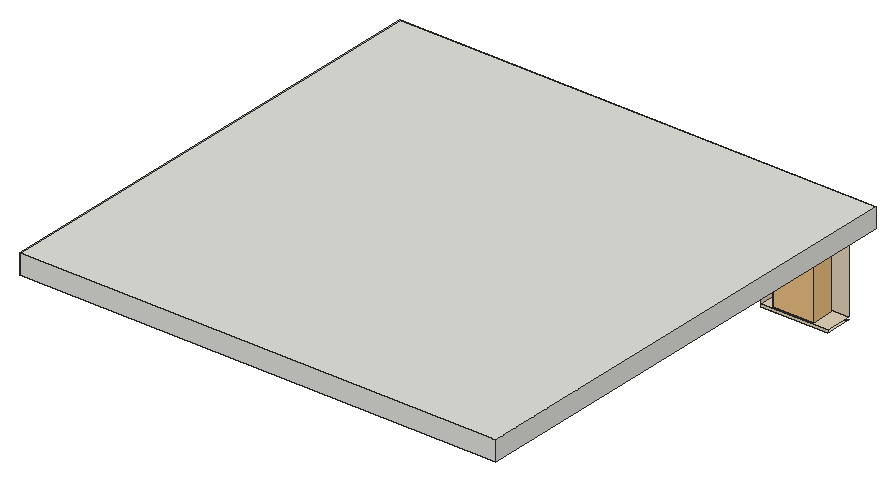
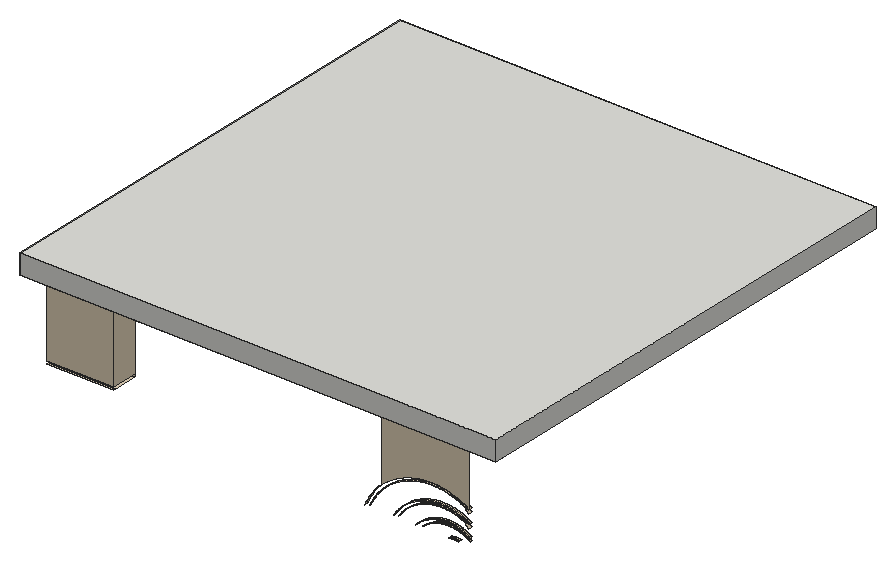
# SketchUp Ruby script. Lengths in inches.
U = 1.inch
M = Sketchup.active_model
def pt(a) = Geom::Point3d.new(a.map { |v| v * U })
def face(e, loops, mat)
  f = e.add_face(loops[0].map { |a| pt(a) })
  loops[1..].each { |l| e.add_face(l.map { |a| pt(a) }).erase! }
  f.material = f.back_material = mat if mat
  f
end
# faces: each face lists its corners as indices into pts; further lists are holes
def faces(e, pts, list, mat = nil) = list.each { |f| face(e, (f[0].is_a?(Array) ? f : [f]).map { |l| l.map { |i| pts[i] } }, mat) }
# xy, xz, yz: faces in a plane at the given z, y or x. An outline is a flat list of corners, or four numbers for a rectangle; further outlines are holes
def ring(l) = l.size == 4 ? [[l[0], l[1]], [l[2], l[1]], [l[2], l[3]], [l[0], l[3]]] : l.each_slice(2).to_a
def flat(e, list, mat, &to3) = list.each { |f| face(e, (f[0].is_a?(Array) ? f : [f]).map { |l| ring(l).map { |u, v| to3.(u, v) } }, mat) }
def xy(e, z, list, mat = nil) = flat(e, list, mat) { |x, y| [x, y, z] }
def xz(e, y, list, mat = nil) = flat(e, list, mat) { |x, z| [x, y, z] }
def yz(e, x, list, mat = nil) = flat(e, list, mat) { |y, z| [x, y, z] }
def lines(e, pts, list) = list.each { |a, b| e.add_line(pt(pts[a]), pt(pts[b])) }
# prism: a flat outline (further loops are holes) pulled along v
def prism(e, loops, v, mat = nil)
  f = face(e, loops, mat); d = Geom::Vector3d.new(v.map { |x| x * U })
  f.pushpull(f.normal.samedirection?(d) ? d.length : -d.length)
end
def box(e, o, s, mat = nil) = prism(e, [[o, [o[0] + s[0], o[1], o[2]], [o[0] + s[0], o[1] + s[1], o[2]], [o[0], o[1] + s[1], o[2]]]], [0, 0, s[2]], mat)
def at(x, y, z, deg = 0) = Geom::Transformation.translation(pt([x, y, z])) * Geom::Transformation.rotation(ORIGIN, Z_AXIS, deg.degrees)
def axes(o, x, y, z) = Geom::Transformation.new([*x, 0, *y, 0, *z, 0, *pt(o).to_a, 1])
def part(name) = M.definitions.add(name)
# library, detail: a bought-in or finely detailed component or shape, given as its bounding box
def library(name, o, s) = part(name).tap { |d| box(d.entities, o, s) }
def detail(e, o, s) = box(e.add_group.entities, o, s)
def put(e, d, t, mat = nil) = e.add_instance(d, t).tap { |i| i.material = mat if mat }
def group(e, t, mat = nil) = e.add_group.tap { |g| g.transformation = t; g.material = mat if mat }.entities
root = M.entities
M.materials.add("Teddy_Brim").color = [225, 210, 185]
M.materials.add("[Color M00]1").color = [255, 255, 255]
c1 = library("Telephone 194 013",[-6.23,-3.22,0.01],[12.47,6.44,15])
c2 = part("Group\#159")
detail(c2.entities,[2.83,2.83,12.39],[3.25,3.25,0.24])
g1 = group(c2.entities,at(3.45,3.45,12.51))
xy(g1,0,[[1,0,0.74,0.03,0.5,0.13,0.29,0.29,0.13,0.5,0.03,0.74,0,1,0.03,1.25,0.13,1.49,0.29,1.7,0.5,1.86,0.74,1.96,1,1.99,1.25,1.96,1.49,1.86,1.7,1.7,1.86,1.49,1.96,1.25,1.99,1,1.96,0.74,1.86,0.5,1.7,0.29,1.49,0.13,1.25,0.03]],"[Color M00]1")
xy(root,89.28,[[15.7,138.5,15.89,139.5],[16.26,138.5,16.44,139.5]],"Teddy_Brim")
xy(root,92.11,[[18.02,138.5,18.28,139]],"Teddy_Brim")
xy(root,93.19,[[18.1,138.5,18.37,139.5],[18.37,138.5,18.64,139.5]],"Teddy_Brim")
xy(root,93.61,[[119.125,131.5,139.5,138.79]],"Teddy_Brim")
xy(root,94.39,[[119.125,131.5,139.5,139.5]],"Teddy_Brim")
xy(root,96.38,[[19.92,138.5,20.25,139]],"Teddy_Brim")
xy(root,97.38,[[19.91,138.5,20.26,139.5]],"Teddy_Brim")
xy(root,101.36,[[22.9375,138.5,23.38,139]],"Teddy_Brim")
xy(root,102.36,[[22.93,138.5,23.39,139.5]],"Teddy_Brim")
xy(root,118,[[115.125,131.5,119.125,131.5,119.125,139.5,139.5,139.5,139.5,144,4.5,144,4.5,139.5,8.5,139.5,8.5,137.5,11.5,137.5,11.5,139.5,115.125,139.5]],"Teddy_Brim")
xz(root,131.5,[[119.125,93.61,139.5,94.39]],"Teddy_Brim")
xz(root,139.5,[[119.125,94.39,139.5,118],[37.98,96.48,37.98,118,11.5,118,11.5,99,12.3,99.48,12.7,99.71,13.52,100.13,13.94,100.33,14.37,100.52,14.79,100.71,15.22,100.88,16.1,101.2,16.98,101.48,17.43,101.6,17.875,101.72,18.33,101.83,18.78,101.92,19.24,102.01,19.69,102.09,20.15,102.16,20.61,102.22,21.08,102.26,21.54,102.3,22,102.33,22.46,102.35,22.93,102.36,23.39,102.36,23.86,102.35,24.32,102.33,24.78,102.3,25.25,102.25,25.71,102.2,26.17,102.14,26.625,102.07,27.08,101.99,27.54,101.9,28.44,101.7,28.89,101.58,29.34,101.45,29.78,101.3125,30.22,101.16,30.66,101.01,31.52,100.67,31.95,100.48,32.37,100.29,32.79,100.09,33.2,99.88,33.61,99.66,34.01,99.43,34.41,99.19,34.72,99,34.81,98.95,35.19,98.69,35.58,98.43,35.96,98.16,36.33,97.88,36.69,97.6,37.05,97.3,37.4,97,37.75,96.69]],"Teddy_Brim")
yz(root,119.125,[[131.5,94.39,139.5,118]],"Teddy_Brim")
p = [[14.78,139.5,89.19],[14.6,139.5,89.16],[14.6,138.5,89.16],[14.78,138.5,89.19],[14.97,139.5,89.22],[14.97,138.5,89.22],
  [15.15,139.5,89.24],[15.15,138.5,89.24],[15.33,139.5,89.26],[15.33,138.5,89.26],[17,139.5,89.24],[16.8125,139.5,89.26],
  [16.8125,138.5,89.26],[17,138.5,89.24],[17.18,139.5,89.22],[17.18,138.5,89.22],[17.36,139.5,89.19],[17.36,138.5,89.19],
  [17.55,139.5,89.16],[17.55,138.5,89.16],[25.625,138.5,89.4],[25.625,139,89.4],[25.82,139,89.24],[25.82,138.5,89.24],
  [41.81,138.5,89.6],[41.81,139,89.6],[42,139,89.2],[42,138.5,89.2],[43.1,139.5,89.19],[42.91,139.5,89.62],
  [42.91,138.5,89.62],[43.1,138.5,89.19],[15.52,139.5,89.27],[15.52,138.5,89.27],[15.7,139.5,89.28],[15.7,138.5,89.28],
  [16.07,139.5,89.29],[15.89,139.5,89.28],[15.89,138.5,89.28],[16.07,138.5,89.29],[16.26,139.5,89.28],[16.26,138.5,89.28],
  [16.63,139.5,89.27],[16.44,139.5,89.28],[16.44,138.5,89.28],[16.63,138.5,89.27],[27.56,139.5,89.26],[27.37,139.5,89.45],
  [27.37,138.5,89.45],[27.56,138.5,89.26],[25.42,138.5,89.57],[25.42,139,89.57],[33.01,138.5,89.67],[33.01,139,89.67],
  [33.19,139,89.4],[33.19,138.5,89.4],[34.41,139.5,89.36],[34.22,139.5,89.66],[34.22,138.5,89.66],[34.41,138.5,89.36],
  [27.18,139.5,89.64],[27.18,138.5,89.64],[25.22,138.5,89.72],[25.22,139,89.72],[26.99,139.5,89.83],[26.99,138.5,89.83],
  [41.61,138.5,90],[41.61,139,90],[42.71,139.5,90.04],[42.71,138.5,90.04],[25.01,138.5,89.88],[25.01,139,89.88],
  [32.8125,138.5,89.94],[32.8125,139,89.94],[34.02,139.5,89.95],[34.02,138.5,89.95],[26.79,139.5,90.02],[26.79,138.5,90.02],
  [24.8,138.5,90.03],[24.8,139,90.03],[32.61,138.5,90.21],[32.61,139,90.21],[24.59,138.5,90.17],[24.59,139,90.17],
  [26.58,139.5,90.19],[26.58,138.5,90.19],[33.82,139.5,90.24],[33.82,138.5,90.24],[41.41,138.5,90.39],[41.41,139,90.39],
  [42.51,139.5,90.45],[42.51,138.5,90.45],[11.5,138.9,90.05],[11.5,139,90.05],[11.7,139,90.1875],[11.7,138.5,90.1875],
  [11.5,138.5,90.05],[11.92,139,90.33],[11.92,138.5,90.33],[24.375,138.5,90.31],[24.375,139,90.31],[26.375,139.5,90.37],
  [26.375,138.5,90.37],[32.41,138.5,90.47],[32.41,139,90.47],[33.62,139.5,90.53],[33.62,138.5,90.53],[12.14,139,90.46],
  [12.14,138.5,90.46],[24.15,138.5,90.45],[24.15,139,90.45],[23.93,138.5,90.57],[23.93,139,90.57],[26.17,139.5,90.54],
  [26.17,138.5,90.54],[41.2,138.5,90.78],[41.2,139,90.78],[12.36,139,90.59],[12.36,138.5,90.59],[25.95,139.5,90.71],
  [25.95,138.5,90.71],[32.2,138.5,90.73],[32.2,139,90.73],[33.41,139.5,90.81],[33.41,138.5,90.81],[42.29,139.5,90.86],
  [42.29,138.5,90.86],[12.58,139,90.71],[12.58,138.5,90.71],[23.71,138.5,90.7],[23.71,139,90.7],[12.8125,139,90.83],
  [12.8125,138.5,90.83],[23.48,138.5,90.82],[23.48,139,90.82],[25.73,139.5,90.87],[25.73,138.5,90.87],[31.98,138.5,90.98],
  [31.98,139,90.98],[13.04,139,90.95],[13.04,138.5,90.95],[23.25,138.5,90.93],[23.25,139,90.93],[33.1875,139.5,91.09],
  [33.1875,138.5,91.09],[40.98,138.5,91.16],[40.98,139,91.16],[13.28,139,91.06],[13.28,138.5,91.06],[23.02,138.5,91.04],
  [23.02,139,91.04],[25.51,139.5,91.02],[25.51,138.5,91.02],[42.07,139.5,91.27],[42.07,138.5,91.27],[11.72,139.5,91.15],
  [11.5,139.5,91],[11.5,138.9,91],[11.5,138.5,91],[11.72,138.5,91.15],[22.78,138.5,91.15],[22.78,139,91.15],
  [25.29,139.5,91.17],[25.29,138.5,91.17],[31.76,138.5,91.23],[31.76,139,91.23],[13.51,139,91.16],[13.51,138.5,91.16],
  [22.54,138.5,91.25],[22.54,139,91.25],[32.96,139.5,91.37],[32.96,138.5,91.37],[11.95,139.5,91.3],[11.95,138.5,91.3],
  [13.75,139,91.26],[13.75,138.5,91.26],[22.3,138.5,91.34],[22.3,139,91.34],[25.06,139.5,91.32],[25.06,138.5,91.32],
  [31.53,138.5,91.47],[31.53,139,91.47],[40.75,138.5,91.54],[40.75,139,91.54],[12.18,139.5,91.44],[12.18,138.5,91.44],
  [13.99,139,91.35],[13.99,138.5,91.35],[22.0625,138.5,91.43],[22.0625,139,91.43],[24.83,139.5,91.46],[24.83,138.5,91.46],
  [41.84,139.5,91.67],[41.84,138.5,91.67],[12.42,139.5,91.58],[12.42,138.5,91.58],[14.23,139,91.44],[14.23,138.5,91.44],
  [14.47,139,91.52],[14.47,138.5,91.52],[21.82,138.5,91.52],[21.82,139,91.52],[32.74,139.5,91.64],[32.74,138.5,91.64],
  [14.72,139,91.6],[14.72,138.5,91.6],[21.57,138.5,91.59],[21.57,139,91.59],[24.59,139.5,91.6],[24.59,138.5,91.6],
  [31.3,138.5,91.71],[31.3,139,91.71],[40.51,138.5,91.92],[40.51,139,91.92],[12.65,139.5,91.71],[12.65,138.5,91.71],
  [14.97,139,91.67],[14.97,138.5,91.67],[21.33,138.5,91.67],[21.33,139,91.67],[24.36,139.5,91.73],[24.36,138.5,91.73],
  [32.5,139.5,91.9],[32.5,138.5,91.9],[12.89,139.5,91.83],[12.89,138.5,91.83],[15.22,139,91.74],[15.22,138.5,91.74],
  [15.47,139,91.8],[15.47,138.5,91.8],[20.83,138.5,91.8],[20.83,139,91.8],[21.08,139,91.73],[21.08,138.5,91.73],
  [24.12,139.5,91.85],[24.12,138.5,91.85],[31.07,138.5,91.94],[31.07,139,91.94],[41.6,139.5,92.07],[41.6,138.5,92.07],
  [13.14,139.5,91.96],[13.14,138.5,91.96],[15.72,139,91.86],[15.72,138.5,91.86],[20.58,138.5,91.85],[20.58,139,91.85],
  [15.97,139,91.91],[15.97,138.5,91.91],[16.22,139,91.95],[16.22,138.5,91.95],[19.81,138.5,91.99],[19.81,139,91.99],
  [20.07,139,91.95],[20.07,138.5,91.95],[20.32,139,91.9],[20.32,138.5,91.9],[23.87,139.5,91.97],[23.87,138.5,91.97],
  [30.82,138.5,92.17],[30.82,139,92.17],[32.26,139.5,92.16],[32.26,138.5,92.16],[40.26,138.5,92.29],[40.26,139,92.29],
  [13.38,139.5,92.07],[13.38,138.5,92.07],[16.48,139,91.99],[16.48,138.5,91.99],[16.73,139,92.03],[16.73,138.5,92.03],
  [16.99,139,92.05],[16.99,138.5,92.05],[19.3,138.5,92.05],[19.3,139,92.05],[19.56,139,92.02],[19.56,138.5,92.02],
  [23.63,139.5,92.09],[23.63,138.5,92.09],[13.63,139.5,92.18],[13.63,138.5,92.18],[17.25,139,92.08],[17.25,138.5,92.08],
  [17.5,139,92.09],[17.5,138.5,92.09],[17.76,139,92.1],[17.76,138.5,92.1],[18.02,139,92.11],[18.02,138.5,92.11],
  [18.28,138.5,92.11],[18.28,139,92.11],[18.53,139,92.1],[18.53,138.5,92.1],[18.79,139,92.09],[18.79,138.5,92.09],
  [19.05,139,92.07],[19.05,138.5,92.07],[23.38,139.5,92.2],[23.38,138.5,92.2],[41.35,139.5,92.46],[41.35,138.5,92.46],
  [13.88,139.5,92.29],[13.88,138.5,92.29],[23.13,139.5,92.3],[23.13,138.5,92.3],[30.58,138.5,92.4],[30.58,139,92.4],
  [32.01,139.5,92.41],[32.01,138.5,92.41],[14.13,139.5,92.38],[14.13,138.5,92.38],[22.875,139.5,92.4],[22.875,138.5,92.4],
  [40.01,138.5,92.65],[40.01,139,92.65],[14.38,139.5,92.48],[14.38,138.5,92.48],[22.62,139.5,92.49],[22.62,138.5,92.49],
  [30.33,138.5,92.61],[30.33,139,92.61],[31.76,139.5,92.66],[31.76,138.5,92.66],[14.64,139.5,92.57],[14.64,138.5,92.57],
  [22.37,139.5,92.58],[22.37,138.5,92.58],[41.09,139.5,92.85],[41.09,138.5,92.85],[14.9,139.5,92.65],[14.9,138.5,92.65],
  [15.16,139.5,92.73],[15.16,138.5,92.73],[22.11,139.5,92.66],[22.11,138.5,92.66],[30.07,138.5,92.83],[30.07,139,92.83],
  [39.75,138.5,93.01],[39.75,139,93.01],[15.42,139.5,92.8],[15.42,138.5,92.8],[21.85,139.5,92.74],[21.59,139.5,92.81],
  [21.59,138.5,92.81],[21.85,138.5,92.74],[31.51,139.5,92.91],[31.51,138.5,92.91],[15.68,139.5,92.86],[15.68,138.5,92.86],
  [21.32,139.5,92.87],[21.32,138.5,92.87],[29.8125,138.5,93.04],[29.8125,139,93.04],[40.82,139.5,93.23],[40.82,138.5,93.23],
  [15.95,139.5,92.92],[15.95,138.5,92.92],[16.21,139.5,92.97],[16.21,138.5,92.97],[21.06,139.5,92.93],[20.79,139.5,92.98],
  [20.79,138.5,92.98],[21.06,138.5,92.93],[31.24,139.5,93.14],[31.24,138.5,93.14],[16.48,139.5,93.02],[16.48,138.5,93.02],
  [16.75,139.5,93.06],[16.75,138.5,93.06],[20.53,139.5,93.03],[20.26,139.5,93.07],[20.26,138.5,93.07],[20.53,138.5,93.03],
  [29.55,138.5,93.24],[29.55,139,93.24],[39.48,138.5,93.36],[39.48,139,93.36],[17.02,139.5,93.1],[17.02,138.5,93.1],
  [17.29,139.5,93.13],[17.29,138.5,93.13],[17.56,139.5,93.15],[17.56,138.5,93.15],[19.72,139.5,93.13],[19.45,139.5,93.16],
  [19.45,138.5,93.16],[19.72,138.5,93.13],[19.99,139.5,93.11],[19.99,138.5,93.11],[30.98,139.5,93.375],[30.98,138.5,93.375],
  [17.83,139.5,93.17],[17.83,138.5,93.17],[18.1,139.5,93.19],[18.1,138.5,93.19],[18.91,139.5,93.1875],[18.64,139.5,93.19],
  [18.64,138.5,93.19],[18.91,138.5,93.1875],[19.18,139.5,93.18],[19.18,138.5,93.18],[29.28,138.5,93.43],[29.28,139,93.43],
  [40.55,139.5,93.6],[40.55,138.5,93.6],[29.01,138.5,93.625],[29.01,139,93.625],[30.71,139.5,93.6],[30.71,138.5,93.6],
  [39.21,138.5,93.7],[39.21,139,93.7],[28.73,138.5,93.81],[28.73,139,93.81],[30.43,139.5,93.82],[30.43,138.5,93.82],
  [40.27,139.5,93.97],[40.27,138.5,93.97],[38.92,138.5,94.05],[38.92,139,94.05],[28.45,138.5,93.99],[28.45,139,93.99],
  [30.15,139.5,94.04],[30.15,138.5,94.04],[11.5,139.5,93.86],[12.5,139.5,94.42],[12.5,139,94.42],[12.5,138.5,94.42],
  [11.5,138.5,93.86],[11.5,138.9,93.86],[28.17,138.5,94.16],[28.17,139,94.16],[29.86,139.5,94.25],[29.86,138.5,94.25],
  [38.63,138.5,94.38],[38.63,139,94.38],[39.98,139.5,94.34],[39.98,138.5,94.34],[27.88,138.5,94.33],[27.88,139,94.33],
  [29.57,139.5,94.45],[29.57,138.5,94.45],[27.59,138.5,94.49],[27.59,139,94.49],[39.68,139.5,94.69],[39.68,138.5,94.69],
  [12.59,139,94.47],[12.59,138.5,94.47],[38.34,138.5,94.71],[38.34,139,94.71],[12.89,139,94.63],[12.89,138.5,94.63],
  [27.29,138.5,94.65],[27.29,139,94.65],[29.28,139.5,94.65],[29.28,138.5,94.65],[13.18,139,94.78],[13.18,138.5,94.78],
  [27,138.5,94.79],[27,139,94.79],[28.98,139.5,94.84],[28.98,138.5,94.84],[38.03,138.5,95.03],[38.03,139,95.03],
  [39.38,139.5,95.04],[39.38,138.5,95.04],[13.48,139,94.92],[13.48,138.5,94.92],[26.7,138.5,94.9375],[26.7,139,94.9375],
  [28.68,139.5,95.02],[28.68,138.5,95.02],[13.79,139,95.06],[13.79,138.5,95.06],[26.39,138.5,95.07],[26.39,139,95.07],
  [11.81,139.5,95.18],[11.5,139.5,95],[11.5,138.9,95],[11.5,138.5,95],[11.81,138.5,95.18],[28.375,139.5,95.2],
  [28.375,138.5,95.2],[37.72,138.5,95.34],[37.72,139,95.34],[39.07,139.5,95.39],[39.07,138.5,95.39],[14.09,139,95.1875],
  [14.09,138.5,95.1875],[26.09,138.5,95.2],[26.09,139,95.2],[12.11,139.5,95.35],[12.11,138.5,95.35],[14.4,139,95.3125],
  [14.4,138.5,95.3125],[25.78,138.5,95.32],[25.78,139,95.32],[28.0625,139.5,95.37],[28.0625,138.5,95.37],[14.71,139,95.43],
  [14.71,138.5,95.43],[25.47,138.5,95.44],[25.47,139,95.44],[37.4,138.5,95.65],[37.4,139,95.65],[12.43,139.5,95.52],
  [12.43,138.5,95.52],[15.03,139,95.54],[15.03,138.5,95.54],[25.15,138.5,95.55],[25.15,139,95.55],[27.75,139.5,95.54],
  [27.75,138.5,95.54],[38.75,139.5,95.72],[38.75,138.5,95.72],[12.74,139.5,95.67],[12.74,138.5,95.67],[15.34,139,95.64],
  [15.34,138.5,95.64],[27.43,139.5,95.69],[27.43,138.5,95.69],[15.66,139,95.74],[15.66,138.5,95.74],[24.84,138.5,95.65],
  [24.84,139,95.65],[13.0625,139.5,95.83],[13.0625,138.5,95.83],[15.98,139,95.83],[15.98,138.5,95.83],[24.52,138.5,95.75],
  [24.52,139,95.75],[27.12,139.5,95.84],[27.12,138.5,95.84],[37.08,138.5,95.95],[37.08,139,95.95],[38.42,139.5,96.05],
  [38.42,138.5,96.05],[13.38,139.5,95.97],[13.38,138.5,95.97],[16.3,139,95.91],[16.3,138.5,95.91],[23.875,138.5,95.92],
  [23.875,139,95.92],[24.2,139,95.84],[24.2,138.5,95.84],[26.79,139.5,95.99],[26.79,138.5,95.99],[16.625,139,95.99],
  [16.625,138.5,95.99],[23.55,138.5,96],[23.55,139,96],[13.71,139.5,96.11],[13.71,138.5,96.11],[16.95,139,96.0625],
  [16.95,138.5,96.0625],[23.23,138.5,96.07],[23.23,139,96.07],[26.47,139.5,96.13],[26.47,138.5,96.13],[36.75,138.5,96.25],
  [36.75,139,96.25],[14.04,139.5,96.24],[14.04,138.5,96.24],[17.28,139,96.125],[17.28,138.5,96.125],[17.6,139,96.18],
  [17.6,138.5,96.18],[22.57,138.5,96.1875],[22.57,139,96.1875],[22.9,139,96.13],[22.9,138.5,96.13],[26.14,139.5,96.26],
  [26.14,138.5,96.26],[38.09,139.5,96.38],[38.09,138.5,96.38],[14.37,139.5,96.37],[14.37,138.5,96.37],[17.93,139,96.23],
  [17.93,138.5,96.23],[18.26,139,96.27],[18.26,138.5,96.27],[21.91,138.5,96.28],[21.91,139,96.28],[22.24,139,96.24],
  [22.24,138.5,96.24],[36.41,138.5,96.54],[36.41,139,96.54],[18.59,139,96.31],[18.59,138.5,96.31],[18.93,139,96.34],
  [18.93,138.5,96.34],[19.26,139,96.36],[19.26,138.5,96.36],[20.92,138.5,96.36],[20.92,139,96.36],[21.25,139,96.34],
  [21.25,138.5,96.34],[21.58,139,96.3125],[21.58,138.5,96.3125],[25.81,139.5,96.38],[25.81,138.5,96.38],[14.7,139.5,96.48],
  [14.7,138.5,96.48],[19.59,139,96.37],[19.59,138.5,96.37],[19.92,139,96.38],[19.92,138.5,96.38],[20.25,138.5,96.38],
  [20.25,139,96.38],[20.59,139,96.375],[20.59,138.5,96.375],[25.47,139.5,96.5],[25.47,138.5,96.5],[37.98,139.5,96.48],
  [37.75,139.5,96.69],[37.75,138.5,96.69],[15.04,139.5,96.6],[15.04,138.5,96.6],[25.14,139.5,96.61],[25.14,138.5,96.61],
  [36.07,138.5,96.82],[36.07,139,96.82],[15.38,139.5,96.7],[15.38,138.5,96.7],[24.8,139.5,96.71],[24.8,138.5,96.71],
  [15.72,139.5,96.8],[15.72,138.5,96.8],[24.46,139.5,96.81],[24.46,138.5,96.81],[37.4,139.5,97],[37.4,138.5,97],
  [16.06,139.5,96.88],[16.06,138.5,96.88],[24.11,139.5,96.89],[24.11,138.5,96.89],[35.72,138.5,97.09],[35.72,139,97.09],
  [16.4,139.5,96.97],[16.4,138.5,96.97],[23.77,139.5,96.98],[23.77,138.5,96.98],[16.75,139.5,97.04],[16.75,138.5,97.04],
  [17.1,139.5,97.11],[17.1,138.5,97.11],[23.42,139.5,97.05],[23.08,139.5,97.12],[23.08,138.5,97.12],[23.42,138.5,97.05],
  [37.05,139.5,97.3],[37.05,138.5,97.3],[17.45,139.5,97.17],[17.45,138.5,97.17],[22.73,139.5,97.17],[22.73,138.5,97.17],
  [35.36,138.5,97.35],[35.36,139,97.35],[17.8,139.5,97.22],[17.8,138.5,97.22],[18.15,139.5,97.27],[18.15,138.5,97.27],
  [22.38,139.5,97.23],[22.03,139.5,97.27],[22.03,138.5,97.27],[22.38,138.5,97.23],[18.5,139.5,97.3],[18.5,138.5,97.3],
  [18.85,139.5,97.33],[18.85,138.5,97.33],[19.2,139.5,97.36],[19.2,138.5,97.36],[21.32,139.5,97.34],[20.97,139.5,97.36],
  [20.97,138.5,97.36],[21.32,138.5,97.34],[21.68,139.5,97.31],[21.68,138.5,97.31],[36.69,139.5,97.6],[36.69,138.5,97.6],
  [19.56,139.5,97.37],[19.56,138.5,97.37],[19.91,139.5,97.38],[19.91,138.5,97.38],[20.62,139.5,97.375],[20.26,139.5,97.38],
  [20.26,138.5,97.38],[20.62,138.5,97.375],[35,138.5,97.61],[35,139,97.61],[34.64,138.5,97.86],[34.64,139,97.86],
  [36.33,139.5,97.88],[36.33,138.5,97.88],[11.5,139.5,97.85],[12.5,139.5,98.4375],[12.5,139,98.4375],[12.5,138.5,98.4375],
  [11.5,138.5,97.85],[11.5,138.9,97.85],[34.27,138.5,98.1],[34.27,139,98.1],[35.96,139.5,98.16],[35.96,138.5,98.16],
  [34.19,138.5,98.15],[34.19,139,98.15],[33.89,138.5,98.34],[33.89,139,98.34],[35.58,139.5,98.43],[35.58,138.5,98.43],
  [33.51,138.5,98.5625],[33.51,139,98.5625],[12.79,139,98.61],[12.79,138.5,98.61],[35.19,139.5,98.69],[35.19,138.5,98.69],
  [13.18,139,98.83],[13.18,138.5,98.83],[33.125,138.5,98.78],[33.125,139,98.78],[34.81,139.5,98.95],[34.81,138.5,98.95],
  [13.57,139,99.04],[13.57,138.5,99.04],[32.74,138.5,98.99],[32.74,139,98.99],[34.72,139.5,99],[34.72,138.5,99],
  [11.9,139.5,99.24],[11.5,139.5,99],[11.5,138.9,99],[11.5,138.5,99],[11.9,138.5,99.24],[13.97,139,99.23],
  [13.97,138.5,99.23],[32.34,138.5,99.19],[32.34,139,99.19],[34.41,139.5,99.19],[34.41,138.5,99.19],[12.3,139.5,99.48],
  [12.3,138.5,99.48],[14.36,139,99.43],[14.36,138.5,99.43],[31.94,138.5,99.39],[31.94,139,99.39],[34.01,139.5,99.43],
  [34.01,138.5,99.43],[14.77,139,99.61],[14.77,138.5,99.61],[31.54,138.5,99.57],[31.54,139,99.57],[33.61,139.5,99.66],
  [33.61,138.5,99.66],[12.7,139.5,99.71],[12.7,138.5,99.71],[15.18,139,99.78],[15.18,138.5,99.78],[31.13,138.5,99.75],
  [31.13,139,99.75],[13.11,139.5,99.92],[13.11,138.5,99.92],[30.72,138.5,99.91],[30.72,139,99.91],[33.2,139.5,99.88],
  [33.2,138.5,99.88],[15.59,139,99.95],[15.59,138.5,99.95],[13.52,139.5,100.13],[13.52,138.5,100.13],[16,139,100.1],
  [16,138.5,100.1],[30.3125,138.5,100.07],[30.3125,139,100.07],[32.79,139.5,100.09],[32.79,138.5,100.09],[13.94,139.5,100.33],
  [13.94,138.5,100.33],[16.42,139,100.25],[16.42,138.5,100.25],[29.89,138.5,100.22],[29.89,139,100.22],[32.37,139.5,100.29],
  [32.37,138.5,100.29],[16.84,139,100.39],[16.84,138.5,100.39],[29.47,138.5,100.36],[29.47,139,100.36],[14.37,139.5,100.52],
  [14.37,138.5,100.52],[31.95,139.5,100.48],[31.95,138.5,100.48],[17.26,139,100.52],[17.26,138.5,100.52],[29.05,138.5,100.49],
  [29.05,139,100.49],[14.79,139.5,100.71],[14.79,138.5,100.71],[17.6875,139,100.64],[17.6875,138.5,100.64],[28.625,138.5,100.61],
  [28.625,139,100.61],[31.52,139.5,100.67],[31.52,138.5,100.67],[18.12,139,100.75],[18.12,138.5,100.75],[28.2,138.5,100.73],
  [28.2,139,100.73],[15.22,139.5,100.88],[15.22,138.5,100.88],[18.55,139,100.85],[18.55,138.5,100.85],[27.77,138.5,100.83],
  [27.77,139,100.83],[31.09,139.5,100.84],[31.09,138.5,100.84],[27.33,138.5,100.93],[27.33,139,100.93],[30.66,139.5,101.01],
  [30.66,138.5,101.01],[15.66,139.5,101.04],[15.66,138.5,101.04],[18.98,139,100.94],[18.98,138.5,100.94],[19.42,139,101.03],
  [19.42,138.5,101.03],[26.9,138.5,101.01],[26.9,139,101.01],[16.1,139.5,101.2],[16.1,138.5,101.2],[19.85,139,101.1],
  [19.85,138.5,101.1],[26.46,138.5,101.09],[26.46,139,101.09],[30.22,139.5,101.16],[30.22,138.5,101.16],[20.29,139,101.17],
  [20.29,138.5,101.17],[26.03,138.5,101.15],[26.03,139,101.15],[16.54,139.5,101.34],[16.54,138.5,101.34],[20.73,139,101.22],
  [20.73,138.5,101.22],[21.17,139,101.27],[21.17,138.5,101.27],[25.15,138.5,101.26],[25.15,139,101.26],[25.59,139,101.21],
  [25.59,138.5,101.21],[29.78,139.5,101.3125],[29.78,138.5,101.3125],[16.98,139.5,101.48],[16.98,138.5,101.48],[21.61,139,101.31],
  [21.61,138.5,101.31],[22.05,139,101.33],[22.05,138.5,101.33],[22.49,139,101.35],[22.49,138.5,101.35],[23.38,138.5,101.36],
  [23.38,139,101.36],[23.82,139,101.35],[23.82,138.5,101.35],[24.26,139,101.33],[24.26,138.5,101.33],[24.71,139,101.3],
  [24.71,138.5,101.3],[29.34,139.5,101.45],[29.34,138.5,101.45],[22.9375,139,101.36],[22.9375,138.5,101.36],[28.89,139.5,101.58],
  [28.89,138.5,101.58],[17.43,139.5,101.6],[17.43,138.5,101.6],[17.875,139.5,101.72],[17.875,138.5,101.72],[28.44,139.5,101.7],
  [28.44,138.5,101.7],[18.33,139.5,101.83],[18.33,138.5,101.83],[27.99,139.5,101.8],[27.99,138.5,101.8],[18.78,139.5,101.92],
  [18.78,138.5,101.92],[27.54,139.5,101.9],[27.54,138.5,101.9],[19.24,139.5,102.01],[19.24,138.5,102.01],[27.08,139.5,101.99],
  [27.08,138.5,101.99],[19.69,139.5,102.09],[19.69,138.5,102.09],[26.625,139.5,102.07],[26.625,138.5,102.07],[20.15,139.5,102.16],
  [20.15,138.5,102.16],[26.17,139.5,102.14],[25.71,139.5,102.2],[25.71,138.5,102.2],[26.17,138.5,102.14],[20.61,139.5,102.22],
  [20.61,138.5,102.22],[21.08,139.5,102.26],[21.08,138.5,102.26],[25.25,139.5,102.25],[25.25,138.5,102.25],[21.54,139.5,102.3],
  [21.54,138.5,102.3],[22,139.5,102.33],[22,138.5,102.33],[22.46,139.5,102.35],[22.46,138.5,102.35],[22.93,139.5,102.36],
  [22.93,138.5,102.36],[23.86,139.5,102.35],[23.39,139.5,102.36],[23.39,138.5,102.36],[23.86,138.5,102.35],[24.32,139.5,102.33],
  [24.32,138.5,102.33],[24.78,139.5,102.3],[24.78,138.5,102.3]]
faces(root,p,[[0,1,2,3],[4,0,3,5],[6,4,5,7],[8,6,7,9],[10,11,12,13],[14,10,13,15],[16,14,15,17],[18,16,17,19],
  [20,21,22,23],[24,25,26,27],[28,29,30,31],[32,8,9,33],[34,32,33,35],[36,37,38,39],[40,36,39,41],[42,43,44,45],
  [11,42,45,12],[46,47,48,49],[50,51,21,20],[52,53,54,55],[56,57,58,59],[47,60,61,48],[62,63,51,50],[60,64,65,61],
  [66,67,25,24],[29,68,69,30],[70,71,63,62],[72,73,53,52],[57,74,75,58],[64,76,77,65],[78,79,71,70],[80,81,73,72],
  [82,83,79,78],[76,84,85,77],[74,86,87,75],[88,89,67,66],[68,90,91,69],[92,93,94,95,96],[95,94,97,98],[99,100,83,82],
  [84,101,102,85],[103,104,81,80],[86,105,106,87],[98,97,107,108],[109,110,100,99],[111,112,110,109],[101,113,114,102],[115,116,89,88],
  [108,107,117,118],[113,119,120,114],[121,122,104,103],[105,123,124,106],[90,125,126,91],[118,117,127,128],[129,130,112,111],[128,127,131,132],
  [133,134,130,129],[119,135,136,120],[137,138,122,121],[132,131,139,140],[141,142,134,133],[123,143,144,124],[145,146,116,115],[140,139,147,148],
  [149,150,142,141],[135,151,152,136],[125,153,154,126],[155,156,157,158,159],[160,161,150,149],[151,162,163,152],[164,165,138,137],[148,147,166,167],
  [168,169,161,160],[143,170,171,144],[172,155,159,173],[167,166,174,175],[176,177,169,168],[162,178,179,163],[180,181,165,164],[182,183,146,145],
  [184,172,173,185],[175,174,186,187],[188,189,177,176],[178,190,191,179],[153,192,193,154],[194,184,185,195],[187,186,196,197],[197,196,198,199],
  [200,201,189,188],[170,202,203,171],[199,198,204,205],[206,207,201,200],[190,208,209,191],[210,211,181,180],[212,213,183,182],[214,194,195,215],
  [205,204,216,217],[218,219,207,206],[208,220,221,209],[202,222,223,203],[224,214,215,225],[217,216,226,227],[227,226,228,229],[230,231,232,233],
  [233,232,219,218],[220,234,235,221],[236,237,211,210],[192,238,239,193],[240,224,225,241],[229,228,242,243],[244,245,231,230],[243,242,246,247],
  [247,246,248,249],[250,251,252,253],[253,252,254,255],[255,254,245,244],[234,256,257,235],[258,259,237,236],[222,260,261,223],[262,263,213,212],
  [264,240,241,265],[249,248,266,267],[267,266,268,269],[269,268,270,271],[272,273,274,275],[275,274,251,250],[256,276,277,257],[278,264,265,279],
  [271,270,280,281],[281,280,282,283],[283,282,284,285],[285,284,286,287],[288,289,290,291],[291,290,292,293],[293,292,294,295],[295,294,273,272],
  [276,296,297,277],[238,298,299,239],[300,278,279,301],[296,302,303,297],[304,305,259,258],[260,306,307,261],[308,300,301,309],[302,310,311,303],
  [312,313,263,262],[314,308,309,315],[310,316,317,311],[318,319,305,304],[306,320,321,307],[322,314,315,323],[316,324,325,317],[298,326,327,299],
  [328,322,323,329],[330,328,329,331],[324,332,333,325],[334,335,319,318],[336,337,313,312],[338,330,331,339],[340,341,342,343],[332,340,343,333],
  [320,344,345,321],[346,338,339,347],[341,348,349,342],[350,351,335,334],[326,352,353,327],[354,346,347,355],[356,354,355,357],[358,359,360,361],
  [348,358,361,349],[344,362,363,345],[364,356,357,365],[366,364,365,367],[368,369,370,371],[359,368,371,360],[372,373,351,350],[374,375,337,336],
  [376,366,367,377],[378,376,377,379],[380,378,379,381],[382,383,384,385],[386,382,385,387],[369,386,387,370],[362,388,389,363],[390,380,381,391],
  [392,390,391,393],[394,395,396,397],[398,394,397,399],[383,398,399,384],[400,401,373,372],[352,402,403,353],[404,405,401,400],[388,406,407,389],
  [408,409,375,374],[410,411,405,404],[406,412,413,407],[402,414,415,403],[416,417,409,408],[418,419,411,410],[412,420,421,413],[422,423,424,425,426,427],
  [428,429,419,418],[420,430,431,421],[432,433,417,416],[414,434,435,415],[436,437,429,428],[430,438,439,431],[440,441,437,436],[434,442,443,435],
  [425,424,444,445],[446,447,433,432],[445,444,448,449],[450,451,441,440],[438,452,453,439],[449,448,454,455],[456,457,451,450],[452,458,459,453],
  [460,461,447,446],[442,462,463,443],[455,454,464,465],[466,467,457,456],[458,468,469,459],[465,464,470,471],[472,473,467,466],[474,475,476,477,478],
  [468,479,480,469],[481,482,461,460],[462,483,484,463],[471,470,485,486],[487,488,473,472],[489,474,478,490],[486,485,491,492],[493,494,488,487],
  [479,495,496,480],[492,491,497,498],[499,500,494,493],[501,502,482,481],[503,489,490,504],[498,497,505,506],[507,508,500,499],[495,509,510,496],
  [483,511,512,484],[513,503,504,514],[506,505,515,516],[509,517,518,510],[516,515,519,520],[521,522,508,507],[523,513,514,524],[520,519,525,526],
  [527,528,522,521],[517,529,530,518],[531,532,502,501],[511,533,534,512],[535,523,524,536],[526,525,537,538],[539,540,541,542],[542,541,528,527],
  [529,543,544,530],[538,537,545,546],[547,548,540,539],[549,535,536,550],[546,545,551,552],[553,554,548,547],[543,555,556,544],[557,558,532,531],
  [559,549,550,560],[552,551,561,562],[562,561,563,564],[565,566,567,568],[568,567,554,553],[555,569,570,556],[533,571,572,534],[573,559,560,574],
  [564,563,575,576],[576,575,577,578],[579,580,581,582],[582,581,566,565],[583,584,558,557],[578,577,585,586],[586,585,587,588],[588,587,589,590],
  [591,592,593,594],[594,593,595,596],[596,595,580,579],[569,597,598,570],[599,573,574,600],[590,589,601,602],[602,601,603,604],[605,606,607,608],
  [608,607,592,591],[597,609,610,598],[571,611,612,613,572],[614,599,600,615],[609,616,617,610],[618,619,584,583],[620,614,615,621],[616,622,623,617],
  [624,620,621,625],[622,626,627,623],[612,628,629,613],[630,624,625,631],[626,632,633,627],[634,635,619,618],[636,630,631,637],[632,638,639,633],
  [640,636,637,641],[642,640,641,643],[644,645,646,647],[638,644,647,639],[628,648,649,629],[650,642,643,651],[645,652,653,646],[654,655,635,634],
  [656,650,651,657],[658,656,657,659],[660,661,662,663],[652,660,663,653],[664,658,659,665],[666,664,665,667],[668,666,667,669],[670,671,672,673],
  [674,670,673,675],[661,674,675,662],[648,676,677,649],[678,668,669,679],[680,678,679,681],[682,683,684,685],[671,682,685,672],[686,687,655,654],
  [688,689,687,686],[676,690,691,677],[692,693,694,695,696,697],[698,699,689,688],[690,700,701,691],[702,703,699,698],[704,705,703,702],[700,706,707,701],
  [708,709,705,704],[695,694,710,711],[706,712,713,707],[711,710,714,715],[716,717,709,708],[712,718,719,713],[715,714,720,721],[722,723,717,716],
  [718,724,725,719],[726,727,728,729,730],[721,720,731,732],[733,734,723,722],[724,735,736,725],[737,726,730,738],[732,731,739,740],[741,742,734,733],
  [735,743,744,736],[740,739,745,746],[747,748,742,741],[743,749,750,744],[751,737,738,752],[746,745,753,754],[755,756,748,747],[757,751,752,758],
  [759,760,756,755],[749,761,762,750],[754,753,763,764],[765,757,758,766],[764,763,767,768],[769,770,760,759],[761,771,772,762],[773,765,766,774],
  [768,767,775,776],[777,778,770,769],[771,779,780,772],[776,775,781,782],[783,784,778,777],[785,773,774,786],[779,787,788,780],[782,781,789,790],
  [791,792,784,783],[793,785,786,794],[790,789,795,796],[797,798,792,791],[787,799,800,788],[796,795,801,802],[803,804,798,797],[805,793,794,806],
  [802,801,807,808],[809,810,804,803],[799,811,812,800],[813,814,810,809],[811,815,816,812],[817,805,806,818],[808,807,819,820],[820,819,821,822],
  [823,824,814,813],[825,817,818,826],[822,821,827,828],[829,830,824,823],[815,831,832,816],[828,827,833,834],[835,836,830,829],[837,825,826,838],
  [834,833,839,840],[840,839,841,842],[843,844,845,846],[846,845,836,835],[831,847,848,832],[849,837,838,850],[842,841,851,852],[852,851,853,854],
  [854,853,855,856],[857,858,859,860],[860,859,861,862],[862,861,863,864],[864,863,844,843],[847,865,866,848],[856,855,867,868],[865,869,870,866],
  [871,849,850,872],[873,871,872,874],[869,875,876,870],[877,873,874,878],[875,879,880,876],[881,877,878,882],[879,883,884,880],[885,881,882,886],
  [883,887,888,884],[889,885,886,890],[887,891,892,888],[893,889,890,894],[895,896,897,898],[891,895,898,892],[899,893,894,900],[901,899,900,902],
  [896,903,904,897],[905,901,902,906],[907,905,906,908],[909,907,908,910],[911,909,910,912],[913,914,915,916],[917,913,916,918],[919,917,918,920],
  [903,919,920,904]],"Teddy_Brim")
g2 = group(root,at(119.125,138.79,93.61),"Teddy_Brim")
xy(g2,0,[[0,0,20.375,0.71]])
put(root,c1,at(128.44,135.43,94.39))
put(root,c2,at(17.05,117.05,105.37))
put(root,c2,at(43.3,117.05,105.37))
put(root,c2,at(69.55,117.05,105.37))
put(root,c2,at(95.8,117.05,105.37))
put(root,c2,at(118.24,117.05,105.37))
put(root,c2,at(118.24,88.05,105.37))
put(root,c2,at(17.05,88.05,105.37))
put(root,c2,at(118.24,59.05,105.37))
put(root,c2,at(17.05,59.05,105.37))
put(root,c2,at(118.24,30.05,105.37))
put(root,c2,at(17.05,30.05,105.37))
put(root,c2,at(118.24,6.55,105.37))
put(root,c2,at(17.05,6.55,105.37))
put(root,c2,at(65.8,6.55,105.37))
put(root,c2,at(92.17,6.55,105.37))
put(root,c2,at(41.67,6.55,105.37))
g3 = group(root,at(0,0,118))
xy(g3,0,[[[0,0,144,144],[4.5,0.95,5.5,0.95,5.5,137.5,138.5,137.5,138.5,0.98,139.5,0.98,139.5,139,4.5,139]]])
xy(g3,6,[[0,0,144,144]])
xz(g3,0,[[0,0,144,6]])
xz(g3,0.95,[[4.5,0,5.5,2]])
xz(g3,0.98,[[138.5,0,139.5,2]])
xz(g3,137.5,[[5.5,0,138.5,2]])
xz(g3,139,[[4.5,0,139.5,2]])
xz(g3,144,[[0,0,144,6]])
yz(g3,0,[[0,0,144,6]])
yz(g3,4.5,[[0.95,0,139,2]])
yz(g3,5.5,[[0.95,0,137.5,2]])
yz(g3,138.5,[[0.98,0,137.5,2]])
yz(g3,139.5,[[0.98,0,139,2]])
yz(g3,144,[[0,0,144,6]])
p = [[5.5,137.5,2],[4.5,137.5,2]]
lines(g3,p,[[0,1]])
g4 = group(g3,at(4.5,0.95,2))
xy(g4,0,[[0,0,1,136.55]])
g5 = group(g3,at(4.5,137.5,2))
xy(g5,0,[[0,0,135,1.5]])
g6 = group(g3,at(138.5,0.98,2))
xy(g6,0,[[0,0,1,136.52]])
